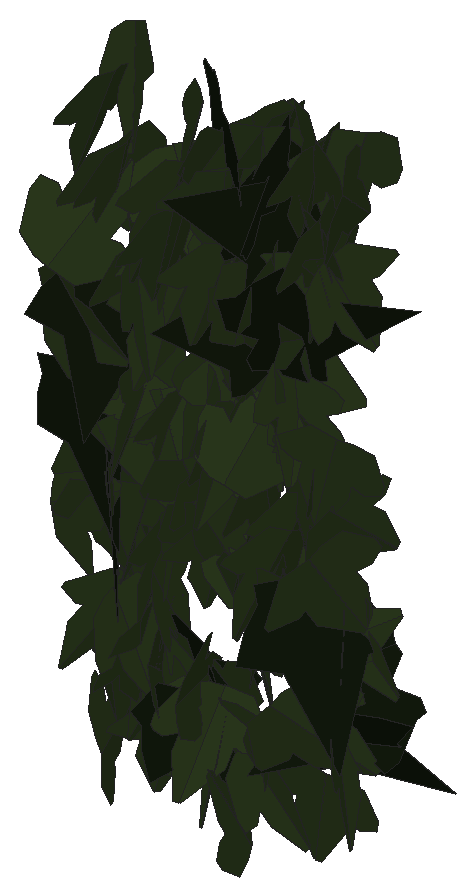
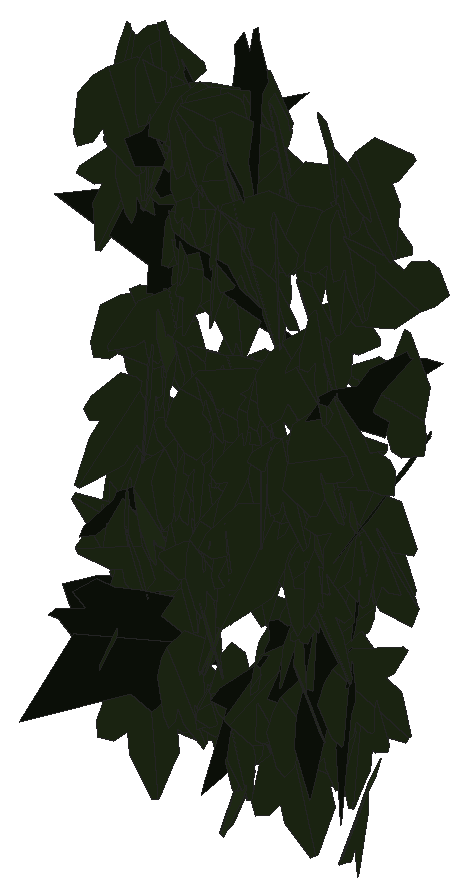
# SketchUp Ruby script. Lengths in inches.
U = 1.inch
M = Sketchup.active_model
def pt(a) = Geom::Point3d.new(a.map { |v| v * U })
def face(e, loops, mat)
  f = e.add_face(loops[0].map { |a| pt(a) })
  loops[1..].each { |l| e.add_face(l.map { |a| pt(a) }).erase! }
  f.material = f.back_material = mat if mat
  f
end
# faces: each face lists its corners as indices into pts; further lists are holes
def faces(e, pts, list, mat = nil) = list.each { |f| face(e, (f[0].is_a?(Array) ? f : [f]).map { |l| l.map { |i| pts[i] } }, mat) }
# xy, xz, yz: faces in a plane at the given z, y or x. An outline is a flat list of corners, or four numbers for a rectangle; further outlines are holes
def ring(l) = l.size == 4 ? [[l[0], l[1]], [l[2], l[1]], [l[2], l[3]], [l[0], l[3]]] : l.each_slice(2).to_a
def flat(e, list, mat, &to3) = list.each { |f| face(e, (f[0].is_a?(Array) ? f : [f]).map { |l| ring(l).map { |u, v| to3.(u, v) } }, mat) }
def xy(e, z, list, mat = nil) = flat(e, list, mat) { |x, y| [x, y, z] }
def xz(e, y, list, mat = nil) = flat(e, list, mat) { |x, z| [x, y, z] }
def yz(e, x, list, mat = nil) = flat(e, list, mat) { |y, z| [x, y, z] }
def lines(e, pts, list) = list.each { |a, b| e.add_line(pt(pts[a]), pt(pts[b])) }
# prism: a flat outline (further loops are holes) pulled along v
def prism(e, loops, v, mat = nil)
  f = face(e, loops, mat); d = Geom::Vector3d.new(v.map { |x| x * U })
  f.pushpull(f.normal.samedirection?(d) ? d.length : -d.length)
end
def box(e, o, s, mat = nil) = prism(e, [[o, [o[0] + s[0], o[1], o[2]], [o[0] + s[0], o[1] + s[1], o[2]], [o[0], o[1] + s[1], o[2]]]], [0, 0, s[2]], mat)
def at(x, y, z, deg = 0) = Geom::Transformation.translation(pt([x, y, z])) * Geom::Transformation.rotation(ORIGIN, Z_AXIS, deg.degrees)
def axes(o, x, y, z) = Geom::Transformation.new([*x, 0, *y, 0, *z, 0, *pt(o).to_a, 1])
def part(name) = M.definitions.add(name)
# library, detail: a bought-in or finely detailed component or shape, given as its bounding box
def library(name, o, s) = part(name).tap { |d| box(d.entities, o, s) }
def detail(e, o, s) = box(e.add_group.entities, o, s)
def put(e, d, t, mat = nil) = e.add_instance(d, t).tap { |i| i.material = mat if mat }
def group(e, t, mat = nil) = e.add_group.tap { |g| g.transformation = t; g.material = mat if mat }.entities
root = M.entities
M.materials.add("efeu1").color = [18, 25, 13]
M.materials.add("efeu2").color = [43, 57, 29]
c1 = part("ivyleaf_9")
p = [[1.54,2.16,1.25],[1.36,2.04,1.19],[-0.21,0.99,0.68],[-0.71,1.11,0.82],[-0.85,0.86,0.67],[-0.8,0.17,0.21],
  [-0.9,-0.01,0.1],[-0.67,-0.16,-0.02],[-0.08,-0.08,-0.05],[-0.03,-0.6,-0.4],[0.65,-0.88,-0.66],[0.83,-0.6,-0.49],
  [1.29,-0.42,-0.43],[1.8125,-0.07,-0.26],[1.21,0.44,0.15]]
faces(c1.entities,p,[[0,1,2,3,4,5,6,7,8,9,10,11,12,13,14]],"efeu1")
c2 = part("ivyleaf_10")
p = [[0,0.5,-0.03],[-0.0625,2.02,-0.43],[-0.19,2.01,-0.46],[-0.54,1.05,-0.29],[-0.52,0.625,-0.18],[-0.83,0.76,-0.28],
  [-1.16,0.64,-0.33],[-1.15,0.33,-0.24],[-0.77,-0.39,0.02],[-0.3,-0.51,0.16],[0.04,-0.48,0.23],[-0.02,2.01,-0.4375],
  [-0.06,2.01,-0.43],[0.04,-0.49,0.23],[0.67,-0.49,0.14],[1.38,0.36,-0.2],[1.375,0.51,-0.24],[0.81,0.65,-0.19],
  [0.62,0.59,-0.15],[0.6,1.09,-0.28],[0.5,1.23,-0.31]]
faces(c2.entities,p,[[0,1,2,3,4,5,6,7,8,9,10],[11,12,0,13,14,15,16,17,18,19,20]],"efeu2")
put(root,c1,axes([519.33,136.34,176.54],[0.02124,-0.04555,-0.77172],[0.73769,-0.22966,0.03386],[-0.23117,-0.73706,0.03715]))
put(root,c2,axes([520.66,136.02,181.65],[-0.00477,-0.71868,-0.00869],[-0.00471,0.00872,-0.71868],[0.71872,-0.00471,-0.00477]))
put(root,c2,axes([520.0625,135.74,175.05],[0.07968,0.69541,0.1918],[-0.00491,0.19348,-0.69948],[-0.72136,0.0755,0.02595]))
put(root,c2,axes([523.81,135.99,178.875],[-0.63522,-0.20678,0.21722],[-0.19628,-0.09804,-0.66731],[0.22675,-0.66413,0.03088]))
put(root,c1,axes([523.37,136.15,176.06],[-0.1268,-0.75891,-0.31784],[0.043,0.31505,-0.76938],[0.82166,-0.1336,-0.00879]))
put(root,c2,axes([523.61,135.85,182.59],[0.03191,-0.68107,-0.2599],[0.03592,0.26131,-0.68033],[0.72809,0.01696,0.04495]))
put(root,c1,axes([522.86,136.4375,182.05],[-0.1549,-0.05537,0.76654],[-0.67702,-0.36023,-0.16284],[0.36371,-0.69412,0.02336]))
put(root,c2,axes([522.52,135.9,181.45],[-0.59963,-0.23915,-0.27782],[0.27864,0.04875,-0.64336],[0.23819,-0.65906,0.05322]))
put(root,c2,axes([522.1875,136.08,180.02],[-0.40597,0.0357,0.61102],[0.61039,-0.03049,0.40734],[0.04517,0.73296,-0.01282]))
put(root,c2,axes([518.64,136.25,176.21],[0.28688,-0.29382,-0.70109],[0.57448,-0.40694,0.40562],[-0.49782,-0.63893,0.06406]))
put(root,c2,axes([523.73,135.73,177.01],[-0.33099,-0.60809,-0.42999],[0.23304,0.36234,-0.69182],[0.70736,-0.40392,0.02672]))
put(root,c2,axes([520.5,136.34,182.09],[0.01748,-0.70092,0.33904],[0.03799,-0.33795,-0.70063],[0.77768,0.03226,0.02661]))
put(root,c2,axes([521.375,136.26,173.19],[0.44095,-0.38423,0.29154],[0.21051,-0.2021,-0.58473],[0.43395,0.48846,-0.0126]))
put(root,c2,axes([523.2,135.75,174.39],[-0.49315,-0.26754,-0.57621],[0.4932,0.29856,-0.56073],[0.40044,-0.6972,-0.019]))
put(root,c2,axes([521.62,136.32,178.36],[0.08956,0.58033,-0.46299],[-0.08299,-0.4556,-0.58712],[-0.73774,0.1217,0.00984]))
put(root,c2,axes([523.87,136.09,173.98],[-0.21618,0.67613,-0.22758],[0.06965,-0.21666,-0.70985],[-0.70999,-0.22713,-0.00034]))
put(root,c2,axes([521.51,136.23,181.18],[-0.21211,-0.64392,0.20108],[-0.04197,-0.19778,-0.67763],[0.67328,-0.21519,0.02111]))
put(root,c2,axes([520.13,135.98,174.58],[0.0262,-0.70373,-0.18372],[0.02742,0.18466,-0.70344],[0.7268,0.0184,0.03316]))
put(root,c1,axes([522.68,135.76,180.54],[0.27282,0.02659,0.75816],[0.75435,0.0759,-0.27411],[-0.08041,0.80217,0.00081]))
put(root,c2,axes([522.41,136.39,176.61],[-0.03261,-0.63607,0.3329],[0.00271,-0.33335,-0.63667],[0.71792,-0.02763,0.01753]))
put(root,c2,axes([521.37,136.23,173.64],[0.54332,0.41778,-0.23532],[-0.18269,-0.14845,-0.68535],[-0.44333,0.57318,-0.00598]))
put(root,c2,axes([518.4375,136.22,179.28],[-0.01464,-0.08882,0.80825],[0.81269,-0.02753,0.0117],[0.02609,0.80791,0.08925]))
put(root,c2,axes([518.92,135.78,180.79],[0.55616,0.25993,-0.47059],[0.38048,0.28805,0.60876],[0.37981,-0.66918,0.07925]))
put(root,c2,axes([521.38,135.62,174.1],[0.06916,0.05618,0.68686],[-0.36134,0.59077,-0.01193],[-0.58683,-0.35715,0.0883]))
put(root,c1,axes([518.7,136.48,177.88],[0.30851,-0.78119,0.124],[0.03261,-0.12042,-0.83979],[0.7903,0.30992,-0.01375]))
put(root,c1,axes([521.8,135.87,183.91],[0.25872,0.00628,-0.71406],[-0.70974,0.08595,-0.2564],[0.07868,0.7546,0.03515]))
put(root,c2,axes([521.94,136.16,180.46],[-0.66714,-0.13294,0.192],[-0.18407,-0.05831,-0.67995],[0.14373,-0.69177,0.02042]))
put(root,c2,axes([522.02,136.27,172.88],[0.33315,-0.06117,0.66451],[0.66709,0.01131,-0.33341],[0.01727,0.74326,0.05976]))
put(root,c2,axes([519.46,136.12,176.55],[-0.70067,-0.17513,-0.1374],[0.13239,0.03694,-0.72221],[0.17895,-0.71305,-0.00367]))
put(root,c2,axes([520.62,135.81,174.27],[-0.15605,0.3068,0.58676],[-0.42018,0.42002,-0.33136],[-0.51173,-0.43843,0.09315]))
put(root,c2,axes([522.61,136.02,181.54],[0.05522,-0.62858,-0.35205],[0.05876,0.35584,-0.62612],[0.71805,0.01922,0.07831]))
put(root,c2,axes([522.22,136.125,176.08],[-0.79796,0.05913,-0.01521],[0.01471,-0.00737,-0.80012],[-0.05925,-0.79807,0.00626]))
put(root,c2,axes([523.46,136.57,182],[0.16281,-0.60948,0.3602],[0.14899,-0.33183,-0.62882],[0.69211,0.21481,0.05063]))
put(root,c2,axes([519.59,136.68,178.14],[0.18749,-0.34717,0.59025],[0.32625,-0.49277,-0.39346],[0.60206,0.37514,0.0294]))
put(root,c2,axes([519.62,136.01,177.07],[-0.27939,0.4503,0.42215],[-0.45374,0.16431,-0.47556],[-0.41845,-0.47882,0.23381]))
put(root,c1,axes([519.1,136.63,179.625],[-0.20645,-0.73431,-0.01218],[0.00174,0.01216,-0.76278],[0.73441,-0.20646,-0.00162]))
put(root,c2,axes([522.02,135.86,178.1875],[0.35464,0.40319,-0.45112],[0.23183,0.39245,0.53299],[0.55886,-0.41864,0.06517]))
put(root,c2,axes([523.28,136.12,182.45],[-0.5777,0.40607,0.05433],[-0.04792,0.02631,-0.70612],[-0.40688,-0.57966,0.00601]))
put(root,c2,axes([519.98,136.26,180.28],[-0.07046,0.69079,-0.11625],[0.02537,-0.11425,-0.69424],[-0.70004,-0.07367,-0.01345]))
put(root,c2,axes([521.32,136.33,181.4375],[0.42127,-0.0179,0.59278],[0.59296,0.02479,-0.42065],[-0.00985,0.7268,0.02895]))
put(root,c2,axes([520.25,136.56,176.05],[0.14373,-0.64063,0.26765],[0.08636,-0.2547,-0.65602],[0.6889,0.16559,0.0264]))
put(root,c2,axes([519.12,136.46,183.14],[0.04784,-0.6977,0.13138],[-0.01249,-0.13249,-0.69902],[0.70986,0.04469,-0.02115]))
put(root,c2,axes([521.48,136.3125,182.41],[-0.40831,-0.56995,0.02167],[-0.0129,-0.01742,-0.70111],[0.57022,-0.40851,-0.00034]))
put(root,c1,axes([522.54,135.8125,182.57],[-0.19868,0.44998,0.63914],[-0.27069,0.57905,-0.49181],[-0.73328,-0.33567,0.00838]))
put(root,c2,axes([523.15,136.37,183.46],[0.06771,-0.74584,-0.01934],[-0.00473,0.01899,-0.7489],[0.74607,0.06781,-0.00299]))
put(root,c2,axes([524.02,135.94,183.28],[0.0956,-0.43647,-0.55522],[-0.04706,0.5551,-0.44448],[0.70468,0.09629,0.04564]))
put(root,c2,axes([522.8,136.34,179.22],[-0.42396,0.08711,-0.54663],[0.5226,-0.16393,-0.43144],[-0.18243,-0.67206,0.03439]))
put(root,c2,axes([520.84,135.94,173.125],[0.21433,0.09598,-0.63414],[0.49539,0.39989,0.22796],[0.40736,-0.53681,0.05643]))
put(root,c2,axes([521.25,136.1875,176.86],[-0.61569,-0.20349,-0.25368],[0.23385,0.10044,-0.64812],[0.226,-0.65829,-0.02047]))
put(root,c2,axes([519.45,136.4,182.1],[0.07795,-0.70977,-0.01957],[0.0004,0.01973,-0.71403],[0.71004,0.07791,0.00255]))
put(root,c2,axes([522.89,136.4,179.61],[0.26735,0.70399,-0.16882],[-0.07992,-0.15016,-0.75276],[-0.71953,0.27826,0.02089]))
put(root,c2,axes([521.57,136.53,171.54],[-0.41466,0.56043,0.30811],[0.14987,-0.27183,0.69614],[0.62173,0.4393,0.03769]))
put(root,c2,axes([520.88,136.34,183.31],[0.40604,-0.57267,-0.17305],[-0.06627,0.1648,-0.70087],[0.59457,0.40946,0.04006]))
put(root,c2,axes([523.35,136.18,183.67],[-0.55468,0.25186,0.41986],[-0.40683,0.11589,-0.60699],[-0.2724,-0.68594,0.05161]))
put(root,c1,axes([520.97,136.15,173.79],[0.07763,-0.4432,-0.62617],[-0.09052,0.61968,-0.44983],[0.76179,0.1188,0.01036]))
put(root,c2,axes([521.06,136.37,178.83],[0.5773,-0.36245,-0.16021],[-0.09425,0.1494,-0.67758],[0.38491,0.5802,0.07439]))
put(root,c2,axes([519.1875,136.75,174.57],[-0.15108,-0.48311,0.45298],[-0.11695,-0.43786,-0.50598],[0.65185,-0.19053,0.01421]))
put(root,c1,axes([522.29,136.37,180.34],[-0.61219,0.27363,0.39767],[-0.36266,0.16314,-0.67056],[-0.31857,-0.71155,-0.00082]))
put(root,c2,axes([520.91,136.32,177.37],[-0.65026,-0.2324,-0.20324],[0.18617,0.08284,-0.69039],[0.24629,-0.67623,-0.01473]))
put(root,c2,axes([523.08,136.24,175.23],[0.34902,0.08698,-0.6989],[0.68429,0.14267,0.35948],[0.16663,-0.76806,-0.01237]))
put(root,c2,axes([522.23,136.73,180.6],[-0.24645,0.21969,-0.6494],[0.43429,-0.48392,-0.32853],[-0.53045,-0.49827,0.03274]))
put(root,c2,axes([521.53,136.49,178.92],[0.68739,-0.01611,-0.14246],[-0.14059,0.06088,-0.68527],[0.02807,0.69936,0.05637]))
put(root,c2,axes([522.49,136.74,177.1],[0.00272,-0.62912,0.27947],[0.05521,-0.27837,-0.62719],[0.68618,0.0249,0.04936]))
put(root,c2,axes([521.68,136.24,178.5],[-0.10509,-0.60885,-0.37772],[0.05116,0.37441,-0.61775],[0.71467,-0.11633,-0.01132]))
put(root,c2,axes([521.42,136.13,182.73],[-0.00513,-0.50341,0.5644],[0.14058,0.55394,0.49536],[-0.7431,0.10827,0.08981]))
put(root,c2,axes([522.49,136.7,173.67],[0.10019,-0.65783,0.16168],[0.02001,-0.1605,-0.66541],[0.67712,0.10208,-0.00426]))
put(root,c2,axes([519.36,136.375,173.82],[-0.637,0.1661,0.16524],[-0.16077,0.03834,-0.65829],[-0.17043,-0.65697,0.00336]))
put(root,c2,axes([521.5625,136.55,178.43],[-0.01498,-0.10325,0.72326],[0.72881,0.04832,0.02199],[-0.05093,0.7218,0.10199]))
put(root,c2,axes([519.75,136.54,173.78],[-0.54693,0.24324,-0.47529],[0.43508,-0.19133,-0.59858],[-0.30947,-0.69888,-0.00155]))
put(root,c2,axes([520.46,136.19,175.39],[-0.2457,0.55479,0.32919],[-0.16396,0.28698,-0.60604],[-0.62392,-0.29389,0.02962]))
put(root,c2,axes([523.7,136.19,181.65],[0.1393,0.60681,0.34219],[-0.03336,0.35438,-0.61484],[-0.69585,0.10449,0.09797]))
put(root,c2,axes([519.18,136.42,177.36],[-0.47309,-0.4131,-0.24707],[0.22107,0.12126,-0.62605],[0.42758,-0.51977,0.05031]))
put(root,c2,axes([519.4,136.45,182.12],[-0.23726,-0.71429,-0.18201],[0.0666,0.16966,-0.7526],[0.7341,-0.24625,0.00945]))
put(root,c2,axes([522.11,136.51,183.27],[-0.61313,-0.34505,-0.01618],[0.0184,0.00029,-0.7035],[0.34494,-0.61334,0.00877]))
put(root,c2,axes([520.11,136.89,173.8],[-0.07236,-0.5682,0.37381],[-0.01204,-0.37479,-0.57202],[0.68003,-0.0671,0.02965]))
put(root,c2,axes([519.78,136.78,176.49],[-0.24175,0.54899,-0.33355],[-0.13382,-0.39161,-0.54756],[-0.62828,-0.12783,0.24497]))
put(root,c2,axes([519.96,136.85,174.43],[0.44457,-0.46319,0.31769],[0.20747,-0.24109,-0.64183],[0.52194,0.49036,-0.01547]))
put(root,c2,axes([521.4,136.49,173.45],[-0.68526,0.02283,0.08212],[-0.08217,-0.00003,-0.68563],[-0.02267,-0.69016,0.00275]))
put(root,c2,axes([522.93,136.93,176.46],[0.27772,-0.47561,0.42894],[0.25432,-0.3472,-0.54963],[0.58781,0.37492,0.03514]))
put(root,c2,axes([522.08,136.46,177.67],[0.02583,-0.65439,-0.26144],[0.03817,0.26253,-0.65335],[0.70365,0.00978,0.04504]))
put(root,c2,axes([521.17,136.68,176.3125],[-0.22658,-0.61865,0.08214],[-0.02932,-0.07673,-0.65884],[0.62339,-0.22847,-0.00114]))
put(root,c2,axes([521.16,136.75,173.51],[-0.55469,-0.10419,-0.43615],[-0.42586,-0.09487,0.56427],[-0.14044,0.69922,0.01157]))
put(root,c2,axes([523.2,136.56,172.82],[-0.68554,-0.14741,0.18921],[-0.18521,-0.0387,-0.70121],[0.15241,-0.71012,-0.00106]))
put(root,c2,axes([520.13,136.91,179.77],[-0.29525,-0.57999,0.3493],[-0.03855,-0.36604,-0.64039],[0.67595,-0.27421,0.11605]))
put(root,c2,axes([521.6,136.59,182.76],[0.2981,-0.63795,-0.19127],[-0.08137,0.1731,-0.70416],[0.66102,0.30901,-0.00042]))
put(root,c2,axes([520.11,136.74,177.97],[-0.62443,-0.09405,-0.24778],[0.26491,-0.24038,-0.57636],[-0.0079,-0.62732,0.258]))
put(root,c2,axes([521.22,136.37,177.5],[-0.2251,-0.5278,-0.44098],[0.1911,0.39773,-0.57358],[0.66069,-0.29486,0.01566]))
put(root,c2,axes([523.18,136.95,175.82],[0.4132,-0.38691,0.46588],[0.3909,-0.26036,-0.56292],[0.46253,0.56568,0.05956]))
put(root,c2,axes([521.71,136.875,182.91],[-0.39579,-0.54105,0.26057],[-0.06755,-0.26997,-0.6632],[0.59671,-0.38943,0.09775]))
put(root,c2,axes([522.45,136.76,177.36],[-0.43297,0.37171,-0.35765],[0.24152,-0.2665,-0.56937],[-0.45579,-0.49432,0.03803]))
put(root,c1,axes([520.24,136.45,174.7],[0.46502,0.17266,-0.58812],[-0.57793,-0.12244,-0.49291],[-0.20421,0.73969,0.05569]))
put(root,c2,axes([523.3125,136.76,175.5],[0.27777,-0.05979,0.6487],[0.65129,0.00986,-0.27797],[0.01444,0.7056,0.05885]))
put(root,c2,axes([519.39,136.62,176.87],[-0.49279,-0.02602,-0.47334],[0.47405,-0.02303,-0.49226],[0.00279,-0.68291,0.03464]))
put(root,c2,axes([523.14,136.49,178.52],[0.29793,-0.53992,-0.35051],[-0.02026,0.37818,-0.59975],[0.6434,0.26192,0.14343]))
put(root,c2,axes([521.75,137.1,178.625],[-0.3175,-0.2365,0.57467],[-0.23015,-0.5547,-0.35543],[0.57725,-0.35123,0.17438]))
put(root,c2,axes([519.13,136.59,178.11],[0.7136,0.0353,-0.13453],[0.13243,0.04244,0.71361],[0.0425,-0.72493,0.03523]))
put(root,c2,axes([520.17,136.8,172.83],[-0.38407,-0.54743,0.12579],[-0.07422,-0.10159,-0.66871],[0.55677,-0.39117,-0.00237]))
put(root,c2,axes([519.61,136.65,180.46],[-0.06798,-0.68485,-0.16919],[0.04407,0.16552,-0.6877],[0.70406,-0.07648,0.02671]))
put(root,c2,axes([523.61,136.38,177.62],[-0.22879,-0.44557,-0.50735],[0.21424,0.4601,-0.50068],[0.64034,-0.31313,-0.01376]))
put(root,c2,axes([521.81,136.63,183.33],[-0.32465,-0.59833,-0.18138],[0.11476,0.14388,-0.68002],[0.6146,-0.34293,0.03117]))
put(root,c2,axes([519.92,136.69,175.98],[0.57255,-0.35955,-0.33793],[-0.28046,0.18876,-0.67601],[0.40597,0.63747,0.00957]))
put(root,c2,axes([520.97,136.52,177.82],[0.36656,-0.46663,-0.37322],[-0.08075,0.39515,-0.57336],[0.59204,0.34281,0.15288]))
put(root,c2,axes([520.79,136.85,180.91],[0.6329,-0.32642,0.00801],[0.00717,-0.00356,-0.71212],[0.32644,0.63294,0.00013]))
put(root,c2,axes([521.7,137.11,176.08],[0.11369,-0.54458,0.41217],[0.16435,-0.38375,-0.55236],[0.6629,0.18854,0.06626]))
put(root,c1,axes([523.77,137.16,174.43],[-0.70293,-0.27658,0.27252],[-0.25409,-0.09853,-0.75538],[0.29361,-0.74744,-0.00127]))
put(root,c2,axes([522.375,136.65,175.86],[-0.52925,0.30414,0.26947],[-0.29221,0.02262,-0.59944],[-0.28237,-0.59348,0.11525]))
put(root,c2,axes([521.86,136.68,175.76],[0.31097,0.62116,0.04643],[-0.04466,-0.02952,0.69414],[0.62129,-0.31303,0.02666]))
put(root,c2,axes([520.32,136.69,182.08],[0.59353,0.38466,0.2506],[0.21106,0.13513,-0.70728],[-0.4077,0.62994,-0.00131]))
put(root,c1,axes([523.37,136.37,173.87],[0.69913,0.28438,0.2271],[0.20777,0.09191,-0.75473],[-0.2988,0.72932,0.00656]))
put(root,c2,axes([519.99,136.71,180.75],[0.47835,-0.42424,-0.32235],[-0.23132,0.22489,-0.63924],[0.47999,0.53118,0.01319]))
put(root,c2,axes([521.64,136.79,174.91],[-0.3601,0.50791,-0.20045],[0.12925,-0.15401,-0.62241],[-0.53052,-0.38227,-0.01558]))
put(root,c2,axes([521.51,136.68,173.33],[0.61263,-0.1376,-0.24836],[-0.18806,0.24588,-0.6001],[0.21273,0.61363,0.18476]))
put(root,c2,axes([519.17,137.01,183.61],[0.59105,-0.2721,0.35994],[0.32776,-0.14878,-0.65067],[0.31011,0.67584,0.00167]))
put(root,c2,axes([522.05,136.96,183.28],[0.08515,-0.70553,0.10179],[0.0189,-0.10024,-0.71062],[0.71258,0.08696,0.00669]))
put(root,c2,axes([521.92,136.98,178.82],[0.54931,-0.26189,0.33521],[0.31996,-0.1064,-0.60745],[0.28031,0.63465,0.03649]))
put(root,c1,axes([519.51,136.48,174.43],[0.25419,-0.00772,-0.71778],[-0.70154,0.15859,-0.25015],[0.15202,0.74477,0.04582]))
put(root,c2,axes([522.33,137.23,179.08],[-0.17052,0.14806,-0.64034],[0.18881,-0.62262,-0.19424],[-0.62953,-0.22684,0.11519]))
put(root,c2,axes([519.26,136.25,172.35],[0.15828,-0.04817,-0.76931],[-0.15596,0.76712,-0.08012],[0.75487,0.16859,0.14476]))
put(root,c2,axes([520.2,136.92,178.09],[0.03024,-0.68133,0.04138],[0.00861,-0.04104,-0.68197],[0.68253,0.03071,0.00677]))
put(root,c2,axes([520.53,136.69,181.5625],[0.27968,-0.6384,-0.28022],[-0.02438,0.29279,-0.69137],[0.69677,0.2665,0.08828]))
put(root,c2,axes([521.55,136.76,176.41],[0.36312,-0.56114,-0.19193],[-0.02634,0.20956,-0.66254],[0.59247,0.35323,0.08817]))
put(root,c2,axes([521.82,136.95,175.26],[0.37202,-0.56833,0.05113],[0.03222,-0.04001,-0.67924],[0.56971,0.37338,0.00503]))
put(root,c2,axes([519.62,137.26,178.5],[-0.03626,0.16976,-0.66055],[-0.37051,-0.56026,-0.12365],[-0.5726,0.35178,0.12183]))
put(root,c2,axes([520.84,136.66,176.52],[-0.51511,-0.48047,-0.32481],[0.25055,0.20745,-0.70419],[0.52305,-0.57254,0.01743]))
put(root,c2,axes([523.41,137.04,183.33],[-0.35036,-0.59755,0.21177],[0.00153,-0.24276,-0.68244],[0.63396,-0.32965,0.11868]))
put(root,c2,axes([521.66,136.68,181.44],[0.20523,-0.61376,-0.3124],[0.02203,0.33166,-0.63713],[0.68834,0.17238,0.11353]))
